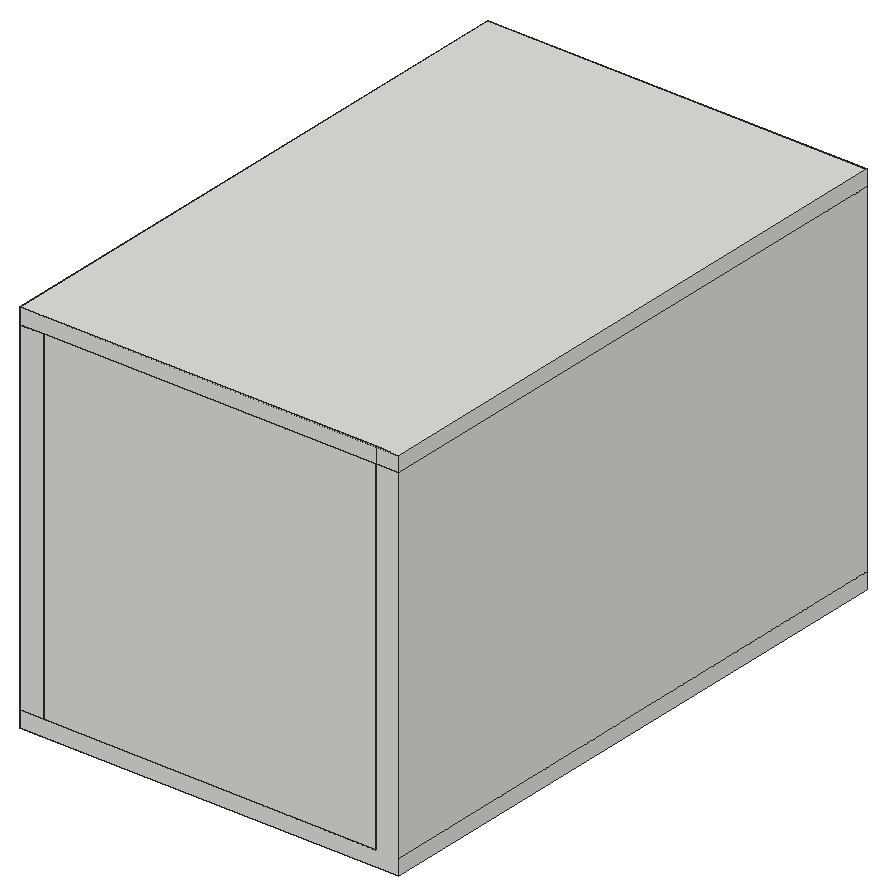
# SketchUp Ruby script. Lengths in inches.
U = 1.inch
M = Sketchup.active_model
def pt(a) = Geom::Point3d.new(a.map { |v| v * U })
def face(e, loops, mat)
  f = e.add_face(loops[0].map { |a| pt(a) })
  loops[1..].each { |l| e.add_face(l.map { |a| pt(a) }).erase! }
  f.material = f.back_material = mat if mat
  f
end
# faces: each face lists its corners as indices into pts; further lists are holes
def faces(e, pts, list, mat = nil) = list.each { |f| face(e, (f[0].is_a?(Array) ? f : [f]).map { |l| l.map { |i| pts[i] } }, mat) }
# xy, xz, yz: faces in a plane at the given z, y or x. An outline is a flat list of corners, or four numbers for a rectangle; further outlines are holes
def ring(l) = l.size == 4 ? [[l[0], l[1]], [l[2], l[1]], [l[2], l[3]], [l[0], l[3]]] : l.each_slice(2).to_a
def flat(e, list, mat, &to3) = list.each { |f| face(e, (f[0].is_a?(Array) ? f : [f]).map { |l| ring(l).map { |u, v| to3.(u, v) } }, mat) }
def xy(e, z, list, mat = nil) = flat(e, list, mat) { |x, y| [x, y, z] }
def xz(e, y, list, mat = nil) = flat(e, list, mat) { |x, z| [x, y, z] }
def yz(e, x, list, mat = nil) = flat(e, list, mat) { |y, z| [x, y, z] }
def lines(e, pts, list) = list.each { |a, b| e.add_line(pt(pts[a]), pt(pts[b])) }
# prism: a flat outline (further loops are holes) pulled along v
def prism(e, loops, v, mat = nil)
  f = face(e, loops, mat); d = Geom::Vector3d.new(v.map { |x| x * U })
  f.pushpull(f.normal.samedirection?(d) ? d.length : -d.length)
end
def box(e, o, s, mat = nil) = prism(e, [[o, [o[0] + s[0], o[1], o[2]], [o[0] + s[0], o[1] + s[1], o[2]], [o[0], o[1] + s[1], o[2]]]], [0, 0, s[2]], mat)
def at(x, y, z, deg = 0) = Geom::Transformation.translation(pt([x, y, z])) * Geom::Transformation.rotation(ORIGIN, Z_AXIS, deg.degrees)
def axes(o, x, y, z) = Geom::Transformation.new([*x, 0, *y, 0, *z, 0, *pt(o).to_a, 1])
def part(name) = M.definitions.add(name)
# library, detail: a bought-in or finely detailed component or shape, given as its bounding box
def library(name, o, s) = part(name).tap { |d| box(d.entities, o, s) }
def detail(e, o, s) = box(e.add_group.entities, o, s)
def put(e, d, t, mat = nil) = e.add_instance(d, t).tap { |i| i.material = mat if mat }
def group(e, t, mat = nil) = e.add_group.tap { |g| g.transformation = t; g.material = mat if mat }.entities
root = M.entities
M.materials.add("Emissive").color = [252, 225, 142]
M.materials.add("Generic").color = [252, 243, 144]
M.materials.add("[Color C05]").color = [203, 169, 125]
c1 = library("cnc 6",[0,0,-0.57],[37.71,74.01,0.57])
c2 = library("pooja copper diya",[482.14,2042.77,132],[4.69,4.76,12.54])
c3 = library("Pooja Unit",[-172.49,-32.78,21.79],[13.09,12.78,4.78])
c4 = library("se",[-3.9,-3.13,0],[7.8,6.26,0.01])
c5 = library("Sphere Light",[-0.98,-0.98,-0.98],[1.96,1.96,1.96])
c6 = library("Group\#22",[0,0,0],[9.33,9.33,26.22])
c7 = library("Group\#324",[0,-0.12,0],[5.27,5.92,4.8])
c8 = library("Lamp Ceiling 35-55",[-2.36,-2.36,-1.36],[4.72,4.72,1.36])
c9 = library("Group\#41",[-0.5,-0.5,0],[92.19,101.19,1.625])
xy(root,-6,[[0,0,144,221.8125]])
xy(root,0,[[9,0,135,170.8125]])
xy(root,2.24,[[9,164.8125,135,170.8125]],"Generic")
xy(root,2.74,[[9.5,164.51,50.5,164.8125],[93.5,164.51,134.5,164.8125]])
xy(root,2.74,[[51.5,164.51,92.5,164.8125]],"Emissive")
xy(root,10.59,[[9.5,164.51,50.5,164.8125],[51.5,164.51,92.5,164.8125],[93.5,164.51,134.5,164.8125]])
xy(root,11.09,[[9,164.8125,135,188.8125]])
xy(root,11.59,[[9.5,188.51,50.5,188.8125],[51.5,188.51,92.5,188.8125],[93.5,188.51,134.5,188.8125]])
xy(root,21.6875,[[9.5,188.51,50.5,188.8125],[51.5,188.51,92.5,188.8125],[93.5,188.51,134.5,188.8125]])
xy(root,22.1875,[[9,188.8125,135,188.8125,135,212.8125,107,212.8125,107,207.8125,106,207.8125,106,212.8125,38,212.8125,38,207.8125,37,207.8125,37,212.8125,9,212.8125]])
xy(root,30.56,[[135,165.3125,140,188.3125]])
xy(root,35.375,[[9,207.8125,37,212.8125],[107,207.8125,135,212.8125]])
xy(root,36.375,[[9,207.8125,37,212.8125],[107,207.8125,135,212.8125]])
xy(root,47.55,[[135,165.3125,140,188.3125]])
xy(root,48.55,[[135,165.3125,140,188.3125]])
xy(root,63.58,[[9,207.8125,37,212.8125],[107,207.8125,135,212.8125]])
xy(root,64.58,[[9,207.8125,37,212.8125],[107,207.8125,135,212.8125]])
xy(root,65.53,[[135,165.3125,140,188.3125]])
xy(root,66.53,[[135,165.3125,140,188.3125]])
xy(root,83.52,[[135,165.3125,140,188.3125]])
xy(root,84.52,[[135,165.3125,140,188.3125]])
xy(root,91.79,[[9,207.8125,37,212.8125],[107,207.8125,135,212.8125]])
xy(root,92.79,[[9,207.8125,37,212.8125],[107,207.8125,135,212.8125]])
xy(root,101.51,[[135,165.3125,140,188.3125]])
xy(root,102.51,[[135,165.3125,140,188.3125]])
xy(root,119.5,[[135,165.3125,140,188.3125]])
xy(root,120,[[37,207.8125,38,212.8125],[106,207.8125,107,212.8125]])
xy(root,131.125,[[0,0,0,221.8125,144,221.8125,144,0,135,0,135,212.8125,9,212.8125,9,0],[9,0,135,212.8125]])
xy(root,137.125,[[0,0,144,221.8125]])
xz(root,0,[[0,-6,144,-6,144,131.125,135,131.125,135,0,0,0],[0,0,9,131.125],[9,0,135,131.125],[0,131.125,135,137.125],[135,131.125,144,137.125]])
xz(root,164.51,[[9.5,2.74,50.5,10.59],[51.5,2.74,92.5,10.59],[93.5,2.74,134.5,10.59]])
xz(root,164.8125,[[[9,2.24,135,11.09],[51.5,2.74,92.5,10.59],[93.5,2.74,134.5,10.59],[9.5,2.74,50.5,10.59]]])
xz(root,165.3125,[[135,30.56,140,47.55],[135,48.55,140,65.53],[135,66.53,140,83.52],[135,84.52,140,101.51],[135,102.51,140,119.5]])
xz(root,170.8125,[[9,0,135,2.24]])
xz(root,188.3125,[[135,30.56,140,47.55],[135,48.55,140,65.53],[135,66.53,140,83.52],[135,84.52,140,101.51],[135,102.51,140,119.5]])
xz(root,188.51,[[9.5,11.59,50.5,21.6875],[51.5,11.59,92.5,21.6875],[93.5,11.59,134.5,21.6875]])
xz(root,188.8125,[[[9,11.09,135,22.1875],[9.5,11.59,50.5,21.6875],[51.5,11.59,92.5,21.6875],[93.5,11.59,134.5,21.6875]]])
xz(root,207.8125,[[37,22.1875,38,22.1875,38,120,37,120,37,92.79,9,92.79,9,91.79,37,91.79,37,64.58,9,64.58,9,63.58,37,63.58,37,36.375,9,36.375,9,35.375,37,35.375],[106,22.1875,107,22.1875,107,35.375,135,35.375,135,36.375,107,36.375,107,63.58,135,63.58,135,64.58,107,64.58,107,91.79,135,91.79,135,92.79,107,92.79,107,120,106,120]])
xz(root,212.8125,[[[38,22.1875,106,120],[72.69,59.73,70.76,59.75,68.83,59.99,66.95,60.42,65.11,61.04,63.36,61.86,61.69,62.85,60.14,64.01,58.72,65.33,57.45,66.79,56.34,68.37,55.39,70.06,54.63,71.84,54.0625,73.69,53.6875,75.59,53.51,77.52,53.54,79.46,53.77,81.38,54.2,83.27,54.83,85.1,55.64,86.86,56.64,88.52,57.8,90.07,59.12,91.49,60.57,92.76,62.16,93.875,63.85,94.82,65.63,95.58,67.48,96.15,69.38,96.53,71.31,96.7,73.24,96.67,75.17,96.4375,77.05,96.01,78.89,95.38,80.64,94.57,82.31,93.58,83.86,92.41,85.28,91.1,86.55,89.64,87.66,88.06,88.61,86.36,89.37,84.58,89.9375,82.73,90.3125,80.83,90.49,78.91,90.46,76.97,90.23,75.05,89.8,73.16,89.17,71.33,88.36,69.57,87.36,67.91,86.2,66.36,84.88,64.9375,83.43,63.66,81.84,62.55,80.15,61.61,78.37,60.84,76.52,60.27,74.62,59.9]],[72.69,59.73,74.62,59.9,76.52,60.27,78.37,60.84,80.15,61.61,81.84,62.55,83.43,63.66,84.88,64.9375,86.2,66.36,87.36,67.91,88.36,69.57,89.17,71.33,89.8,73.16,90.23,75.05,90.46,76.97,90.49,78.91,90.3125,80.83,89.9375,82.73,89.37,84.58,88.61,86.36,87.66,88.06,86.55,89.64,85.28,91.1,83.86,92.41,82.31,93.58,80.64,94.57,78.89,95.38,77.05,96.01,75.17,96.4375,73.24,96.67,71.31,96.7,69.38,96.53,67.48,96.15,65.63,95.58,63.85,94.82,62.16,93.875,60.57,92.76,59.12,91.49,57.8,90.07,56.64,88.52,55.64,86.86,54.83,85.1,54.2,83.27,53.77,81.38,53.54,79.46,53.51,77.52,53.6875,75.59,54.0625,73.69,54.63,71.84,55.39,70.06,56.34,68.37,57.45,66.79,58.72,65.33,60.14,64.01,61.69,62.85,63.36,61.86,65.11,61.04,66.95,60.42,68.83,59.99,70.76,59.75],[9,120,135,131.125]])
xz(root,212.8125,[[9,64.58,37,91.79],[107,64.58,135,91.79]],"Emissive")
xz(root,212.8125,[[9,22.1875,37,35.375],[107,22.1875,135,35.375],[9,36.375,37,63.58],[107,36.375,135,63.58],[9,92.79,37,120],
  [107,92.79,135,120]],"Generic")
xz(root,221.8125,[[0,-6,144,0],[0,0,144,120],[0,120,144,131.125],[0,131.125,144,137.125]])
yz(root,0,[[0,-6,221.8125,0],[0,0,221.8125,131.125],[0,131.125,221.8125,137.125]])
yz(root,9,[[0,0,170.8125,0,170.8125,2.24,164.8125,2.24,164.8125,11.09,188.8125,11.09,188.8125,22.1875,212.8125,22.1875,212.8125,35.375,207.8125,35.375,207.8125,36.375,212.8125,36.375,212.8125,63.58,207.8125,63.58,207.8125,64.58,212.8125,64.58,212.8125,91.79,207.8125,91.79,207.8125,92.79,212.8125,92.79,212.8125,131.125,0,131.125]])
yz(root,9.5,[[164.51,2.74,164.8125,10.59],[188.51,11.59,188.8125,21.6875]])
yz(root,37,[[207.8125,22.1875,212.8125,35.375],[207.8125,36.375,212.8125,63.58],[207.8125,64.58,212.8125,91.79],[207.8125,92.79,212.8125,120]])
yz(root,38,[[207.8125,22.1875,212.8125,120]],"Generic")
yz(root,50.5,[[164.51,2.74,164.8125,10.59],[188.51,11.59,188.8125,21.6875]])
yz(root,51.5,[[164.51,2.74,164.8125,10.59],[188.51,11.59,188.8125,21.6875]])
yz(root,92.5,[[164.51,2.74,164.8125,10.59],[188.51,11.59,188.8125,21.6875]])
yz(root,93.5,[[164.51,2.74,164.8125,10.59],[188.51,11.59,188.8125,21.6875]])
yz(root,106,[[207.8125,22.1875,212.8125,120]],"Generic")
yz(root,107,[[207.8125,22.1875,212.8125,35.375],[207.8125,36.375,212.8125,63.58],[207.8125,64.58,212.8125,91.79],[207.8125,92.79,212.8125,120]])
yz(root,134.5,[[164.51,2.74,164.8125,10.59],[188.51,11.59,188.8125,21.6875]])
yz(root,135,[[0,0,0,131.125,212.8125,131.125,212.8125,120,164.8125,120,164.8125,30.06,188.8125,30.06,188.8125,120,212.8125,120,212.8125,92.79,207.8125,92.79,207.8125,91.79,212.8125,91.79,212.8125,64.58,207.8125,64.58,207.8125,63.58,212.8125,63.58,212.8125,36.375,207.8125,36.375,207.8125,35.375,212.8125,35.375,212.8125,22.1875,188.8125,22.1875,188.8125,11.09,164.8125,11.09,164.8125,2.24,170.8125,2.24,170.8125,0],[[164.8125,30.06,188.8125,120],[165.3125,102.51,188.3125,119.5],[165.3125,84.52,188.3125,101.51],[165.3125,48.55,188.3125,65.53],[165.3125,30.56,188.3125,47.55],[165.3125,66.53,188.3125,83.52]]])
yz(root,140,[[165.3125,30.56,188.3125,47.55],[165.3125,48.55,188.3125,65.53],[165.3125,66.53,188.3125,83.52],[165.3125,84.52,188.3125,101.51],[165.3125,102.51,188.3125,119.5]])
yz(root,144,[[0,-6,221.8125,0],[0,0,221.8125,131.125],[0,131.125,221.8125,137.125]])
p = [[-131.24,-227.08,34.42],[-131.31,-226.76,35.41],[-131.31,-226.74,35.41]]
lines(root,p,[[0,1],[2,0]])
put(root,c1,axes([37,212.02,120],[-0.7439,0,0],[0,0,-0.36765],[0,-0.27,0]))
put(root,c1,axes([37,212.22,91.79],[-0.74258,0,0],[0,0,-0.36765],[0,-0.27,0]))
put(root,c1,axes([37,212.125,63.58],[-0.74258,0,0],[0,0,-0.36765],[0,-0.27,0]))
put(root,c1,axes([135,212.5625,63.58],[-0.74258,0,0],[0,0,-0.36765],[0,-0.27,0]))
put(root,c1,axes([135,212.3125,91.79],[-0.74258,0,0],[0,0,-0.36624],[0,-0.27,0]))
put(root,c1,axes([135,211.76,119.79],[-0.74258,0,0],[0,0,-0.36483],[0,-0.27,0]))
put(root,c2,axes([-917.71,-3886.58,-241.8125],[2,0,0],[0,2,0],[0,0,2]))
put(root,c2,axes([-871.77,-3880.73,-241.8125],[2,0,0],[0,2,0],[0,0,2]))
put(root,c1,axes([135,212.8125,33.95],[-0.74258,0,0],[0,0,-0.16059],[0,0.16733,0]))
put(root,c1,axes([37,212.19,36.9],[-0.73189,0,0],[0,0,-0.20588],[0,-0.1512,0]))
put(root,c3,at(233.31,225.98,0))
put(root,c4,axes([75.3,164.51,5.04],[0.47462,0,0],[0,0,0.47462],[0,-0.47462,0]))
put(root,c4,axes([26.55,164.51,5.04],[0.47462,0,0],[0,0,0.47462],[0,-0.47462,0]))
put(root,c4,axes([114.36,164.51,5.04],[0.47462,0,0],[0,0,0.47462],[0,-0.47462,0]))
put(root,c4,axes([120.24,188.51,15.39],[0.47462,0,0],[0,0,0.47462],[0,-0.47462,0]))
put(root,c4,axes([70.86,188.51,15.39],[0.47462,0,0],[0,0,0.47462],[0,-0.47462,0]))
put(root,c4,axes([31.86,188.51,15.39],[0.47462,0,0],[0,0,0.47462],[0,-0.47462,0]))
put(root,c5,at(136.74,178.09,119.5))
put(root,c5,at(139.02,176.23,101.52))
put(root,c5,at(139.02,176.23,83.52))
put(root,c5,at(139.02,176.23,65.58))
put(root,c5,at(139.02,178.1,47.37))
g1 = group(root,at(128.4,212,22.1875,90))
xy(g1,0,[[0,0,0.72,8.36]],"[Color C05]")
xy(g1,0.24,[[0,0.24,0.36,8.12],[0.36,0.24,0.72,8.12]],"[Color C05]")
xy(g1,11.07,[[0,0.24,0.36,8.12],[0.36,0.24,0.72,8.12]],"[Color C05]")
xy(g1,11.3125,[[0,0,0.72,8.36]],"[Color C05]")
xz(g1,0,[[0,0,0.72,11.3125]],"[Color C05]")
xz(g1,0.24,[[0,0.24,0.36,11.07],[0.36,0.24,0.72,11.07]],"[Color C05]")
xz(g1,8.12,[[0,0.24,0.36,11.07],[0.36,0.24,0.72,11.07]],"[Color C05]")
xz(g1,8.36,[[0,0,0.72,11.3125]],"[Color C05]")
yz(g1,0,[[[0,0,8.36,11.3125],[0.24,0.24,8.12,11.07]]],"[Color C05]")
yz(g1,0.36,[[[0.24,0.24,8.12,11.07],[1.2,1.2,7.16,10.11]]])
yz(g1,0.72,[[[0,0,8.36,11.3125],[0.24,0.24,8.12,11.07]]],"[Color C05]")
g2 = group(root,at(129,207.5,93.54))
xy(g2,0,[[-12.04,0,0,1.04]],"[Color C05]")
xy(g2,0.34,[[-11.7,0,-0.34,0.52],[-11.7,0.52,-0.34,1.04]],"[Color C05]")
xy(g2,15.94,[[-11.7,0,-0.34,0.52],[-11.7,0.52,-0.34,1.04]],"[Color C05]")
xy(g2,16.29,[[-12.04,0,0,1.04]],"[Color C05]")
xz(g2,0,[[[-12.04,0,0,16.29],[-11.7,0.34,-0.34,15.94]]],"[Color C05]")
xz(g2,0.52,[[[-11.7,0.34,-0.34,15.94],[-10.32,1.72,-1.72,14.56]]])
xz(g2,1.04,[[[-12.04,0,0,16.29],[-11.7,0.34,-0.34,15.94]]],"[Color C05]")
yz(g2,-12.04,[[0,0,1.04,16.29]],"[Color C05]")
yz(g2,-11.7,[[0,0.34,0.52,15.94],[0.52,0.34,1.04,15.94]],"[Color C05]")
yz(g2,-0.34,[[0,0.34,0.52,15.94],[0.52,0.34,1.04,15.94]],"[Color C05]")
yz(g2,0,[[0,0,1.04,16.29]],"[Color C05]")
g3 = group(root,at(30.24,209.94,22.39))
xy(g3,0,[[-9.36,0,0,0.81]],"[Color C05]")
xy(g3,0.27,[[-9.1,0,-0.27,0.4],[-9.1,0.4,-0.27,0.81]],"[Color C05]")
xy(g3,12.4,[[-9.1,0,-0.27,0.4],[-9.1,0.4,-0.27,0.81]],"[Color C05]")
xy(g3,12.67,[[-9.36,0,0,0.81]],"[Color C05]")
xz(g3,0,[[[-9.36,0,0,12.67],[-9.1,0.27,-0.27,12.4]]],"[Color C05]")
xz(g3,0.4,[[[-9.1,0.27,-0.27,12.4],[-8.02,1.34,-1.34,11.33]]])
xz(g3,0.81,[[[-9.36,0,0,12.67],[-9.1,0.27,-0.27,12.4]]],"[Color C05]")
yz(g3,-9.36,[[0,0,0.81,12.67]],"[Color C05]")
yz(g3,-9.1,[[0,0.27,0.4,12.4],[0.4,0.27,0.81,12.4]],"[Color C05]")
yz(g3,-0.27,[[0,0.27,0.4,12.4],[0.4,0.27,0.81,12.4]],"[Color C05]")
yz(g3,0,[[0,0,0.81,12.67]],"[Color C05]")
g4 = group(root,at(28.8125,210.59,92.79))
xy(g4,0,[[-12.14,0,0,1.04]],"[Color C05]")
xy(g4,0.35,[[-11.79,0,-0.35,0.52],[-11.79,0.52,-0.35,1.04]],"[Color C05]")
xy(g4,16.07,[[-11.79,0,-0.35,0.52],[-11.79,0.52,-0.35,1.04]],"[Color C05]")
xy(g4,16.42,[[-12.14,0,0,1.04]],"[Color C05]")
xz(g4,0,[[[-12.14,0,0,16.42],[-11.79,0.35,-0.35,16.07]]],"[Color C05]")
xz(g4,0.52,[[[-11.79,0.35,-0.35,16.07],[-10.4,1.74,-1.74,14.68]]])
xz(g4,1.04,[[[-12.14,0,0,16.42],[-11.79,0.35,-0.35,16.07]]],"[Color C05]")
yz(g4,-12.14,[[0,0,1.04,16.42]],"[Color C05]")
yz(g4,-11.79,[[0,0.35,0.52,16.07],[0.52,0.35,1.04,16.07]],"[Color C05]")
yz(g4,-0.35,[[0,0.35,0.52,16.07],[0.52,0.35,1.04,16.07]],"[Color C05]")
yz(g4,0,[[0,0,1.04,16.42]],"[Color C05]")
g5 = group(root,at(128.43,211.56,36.375))
xy(g5,0,[[-11.71,0,0,1.01]],"[Color C05]")
xy(g5,0.34,[[-11.37,0,-0.34,0.5],[-11.37,0.5,-0.34,1.01]],"[Color C05]")
xy(g5,15.5,[[-11.37,0,-0.34,0.5],[-11.37,0.5,-0.34,1.01]],"[Color C05]")
xy(g5,15.84,[[-11.71,0,0,1.01]],"[Color C05]")
xz(g5,0,[[[-11.71,0,0,15.84],[-11.37,0.34,-0.34,15.5]]],"[Color C05]")
xz(g5,0.5,[[[-11.37,0.34,-0.34,15.5],[-10.03,1.68,-1.68,14.16]]])
xz(g5,1.01,[[[-11.71,0,0,15.84],[-11.37,0.34,-0.34,15.5]]],"[Color C05]")
yz(g5,-11.71,[[0,0,1.01,15.84]],"[Color C05]")
yz(g5,-11.37,[[0,0.34,0.5,15.5],[0.5,0.34,1.01,15.5]],"[Color C05]")
yz(g5,-0.34,[[0,0.34,0.5,15.5],[0.5,0.34,1.01,15.5]],"[Color C05]")
yz(g5,0,[[0,0,1.01,15.84]],"[Color C05]")
g6 = group(root,at(30.17,211.08,64.58))
xy(g6,0,[[-11.79,0,0,1.01]],"[Color C05]")
xy(g6,0.34,[[-11.45,0,-0.34,0.51],[-11.45,0.51,-0.34,1.01]],"[Color C05]")
xy(g6,15.61,[[-11.45,0,-0.34,0.51],[-11.45,0.51,-0.34,1.01]],"[Color C05]")
xy(g6,15.95,[[-11.79,0,0,1.01]],"[Color C05]")
xz(g6,0,[[[-11.79,0,0,15.95],[-11.45,0.34,-0.34,15.61]]],"[Color C05]")
xz(g6,0.51,[[[-11.45,0.34,-0.34,15.61],[-10.1,1.6875,-1.6875,14.26]]])
xz(g6,1.01,[[[-11.79,0,0,15.95],[-11.45,0.34,-0.34,15.61]]],"[Color C05]")
yz(g6,-11.79,[[0,0,1.01,15.95]],"[Color C05]")
yz(g6,-11.45,[[0,0.34,0.51,15.61],[0.51,0.34,1.01,15.61]],"[Color C05]")
yz(g6,-0.34,[[0,0.34,0.51,15.61],[0.51,0.34,1.01,15.61]],"[Color C05]")
yz(g6,0,[[0,0,1.01,15.95]],"[Color C05]")
g7 = group(root,at(30.79,210.99,36.375))
xy(g7,0,[[-12.625,0,0,1.09]],"[Color C05]")
xy(g7,0.36,[[-12.26,0,-0.36,0.54],[-12.26,0.54,-0.36,1.09]],"[Color C05]")
xy(g7,16.72,[[-12.26,0,-0.36,0.54],[-12.26,0.54,-0.36,1.09]],"[Color C05]")
xy(g7,17.08,[[-12.625,0,0,1.09]],"[Color C05]")
xz(g7,0,[[[-12.625,0,0,17.08],[-12.26,0.36,-0.36,16.72]]],"[Color C05]")
xz(g7,0.54,[[[-12.26,0.36,-0.36,16.72],[-10.82,1.81,-1.81,15.27]]])
xz(g7,1.09,[[[-12.625,0,0,17.08],[-12.26,0.36,-0.36,16.72]]],"[Color C05]")
yz(g7,-12.625,[[0,0,1.09,17.08]],"[Color C05]")
yz(g7,-12.26,[[0,0.36,0.54,16.72],[0.54,0.36,1.09,16.72]],"[Color C05]")
yz(g7,-0.36,[[0,0.36,0.54,16.72],[0.54,0.36,1.09,16.72]],"[Color C05]")
yz(g7,0,[[0,0,1.09,17.08]],"[Color C05]")
g8 = group(root,at(127.76,210.97,64.58))
xy(g8,0,[[-9.95,0,0,0.86]],"[Color C05]")
xy(g8,0.29,[[-9.67,0,-0.29,0.43],[-9.67,0.43,-0.29,0.86]],"[Color C05]")
xy(g8,13.18,[[-9.67,0,-0.29,0.43],[-9.67,0.43,-0.29,0.86]],"[Color C05]")
xy(g8,13.46,[[-9.95,0,0,0.86]],"[Color C05]")
xz(g8,0,[[[-9.95,0,0,13.46],[-9.67,0.29,-0.29,13.18]]],"[Color C05]")
xz(g8,0.43,[[[-9.67,0.29,-0.29,13.18],[-8.52,1.43,-1.43,12.04]]])
xz(g8,0.86,[[[-9.95,0,0,13.46],[-9.67,0.29,-0.29,13.18]]],"[Color C05]")
yz(g8,-9.95,[[0,0,0.86,13.46]],"[Color C05]")
yz(g8,-9.67,[[0,0.29,0.43,13.18],[0.43,0.29,0.86,13.18]],"[Color C05]")
yz(g8,-0.29,[[0,0.29,0.43,13.18],[0.43,0.29,0.86,13.18]],"[Color C05]")
yz(g8,0,[[0,0,0.86,13.46]],"[Color C05]")
put(root,c6,axes([58.53,173.26,99.51],[0.8316,0,0],[0,0.8316,0],[0,0,1.13929]))
put(root,c7,axes([134.73,176.93,30.56],[1,0,0],[0,1,0],[0,0,0.59]))
put(root,c7,axes([31.89,207.16,22.1875],[0.55,0,0],[0,0.55,0],[0,0,0.3245]))
put(root,c7,axes([16.83,207.16,22.1875],[0.55,0,0],[0,0.55,0],[0,0,0.3245]))
put(root,c7,axes([15.57,207.8125,36.375],[0.55,0,0],[0,0.55,0],[0,0,0.3245]))
put(root,c7,axes([31.5,207.8125,36.375],[0.55,0,0],[0,0.55,0],[0,0,0.3245]))
put(root,c7,axes([30.13,207.88,64.58],[0.55,0,0],[0,0.55,0],[0,0,0.3245]))
put(root,c7,axes([15.77,207.8125,64.58],[0.55,0,0],[0,0.55,0],[0,0,0.3245]))
put(root,c7,axes([13.5625,207.88,92.79],[0.55,0,0],[0,0.55,0],[0,0,0.3245]))
put(root,c7,axes([29.1875,207.88,92.79],[0.55,0,0],[0,0.55,0],[0,0,0.3245]))
put(root,c7,axes([113.125,207.88,92.79],[0.55,0,0],[0,0.55,0],[0,0,0.3245]))
put(root,c7,axes([130.6875,207.88,92.79],[0.55,0,0],[0,0.55,0],[0,0,0.3245]))
put(root,c7,axes([128.47,207.88,64.58],[0.55,0,0],[0,0.55,0],[0,0,0.3245]))
put(root,c7,axes([112.47,207.88,64.58],[0.55,0,0],[0,0.55,0],[0,0,0.3245]))
put(root,c7,axes([112.47,207.88,36.375],[0.55,0,0],[0,0.55,0],[0,0,0.3245]))
put(root,c7,axes([129.09,207.88,36.375],[0.55,0,0],[0,0.55,0],[0,0,0.3245]))
put(root,c7,axes([129.1,209.06,22.1875],[0.55,0,0],[0,0.55,0],[0,0,0.3245]))
put(root,c7,axes([114.66,209.06,22.1875],[0.55,0,0],[0,0.55,0],[0,0,0.3245]))
put(root,c7,axes([134.73,176.93,48.55],[1,0,0],[0,1,0],[0,0,0.59]))
put(root,c7,axes([134.73,173.85,66.53],[1,0,0],[0,1,0],[0,0,0.59]))
put(root,c7,axes([134.73,173.85,84.78],[1,0,0],[0,1,0],[0,0,0.59]))
put(root,c7,axes([134.73,172.2,102.14],[1,0,0],[0,1,0],[0,0,0.59]))
g9 = group(root,at(9,77.8125,125.77))
xy(g9,0.36,[[[0,0,126,135],[17.68,17.68,108.32,117.32]]])
xy(g9,1.98,[[17.43,17.38,108.62,17.68],[17.43,17.68,17.68,117.57],[108.32,17.68,108.62,117.57],[17.68,117.32,108.32,117.57]])
xy(g9,3.61,[[17.43,17.38,108.62,117.57]])
xy(g9,5.36,[[0,0,126,135]])
xz(g9,0,[[0,0.36,126,5.36]])
xz(g9,17.68,[[17.68,0.36,108.32,1.98]])
xz(g9,117.32,[[17.68,0.36,108.32,1.98]])
xz(g9,135,[[0,0.36,126,5.36]])
yz(g9,0,[[0,0.36,135,5.36]])
yz(g9,17.68,[[17.68,0.36,117.32,1.98]])
yz(g9,108.32,[[17.68,0.36,117.32,1.98]])
yz(g9,126,[[0,0.36,135,5.36]])
put(g9,c8,at(6.08,63.86,1.61))
put(g9,c8,at(62.71,7.85,1.72))
put(g9,c8,at(117.18,110.3125,1.36))
put(g9,c8,at(108.34,8.85,1.55))
put(g9,c8,at(63.24,125.33,1.48))
put(g9,c8,at(117.12,45.24,1.61))
put(g9,c8,at(8.59,112.28,1.55))
put(g9,c8,at(8.05,10.08,1.61))
put(g9,c9,at(17.43,17.38,1.98))
put(root,c6,axes([69.62,172.32,108.1],[0.594,0,0],[0,0.594,0],[0,0,0.81378]))
put(root,c6,axes([83.74,169.9375,98.93],[0.84942,0,0],[0,0.84942,0],[0,0,1.16371]))
